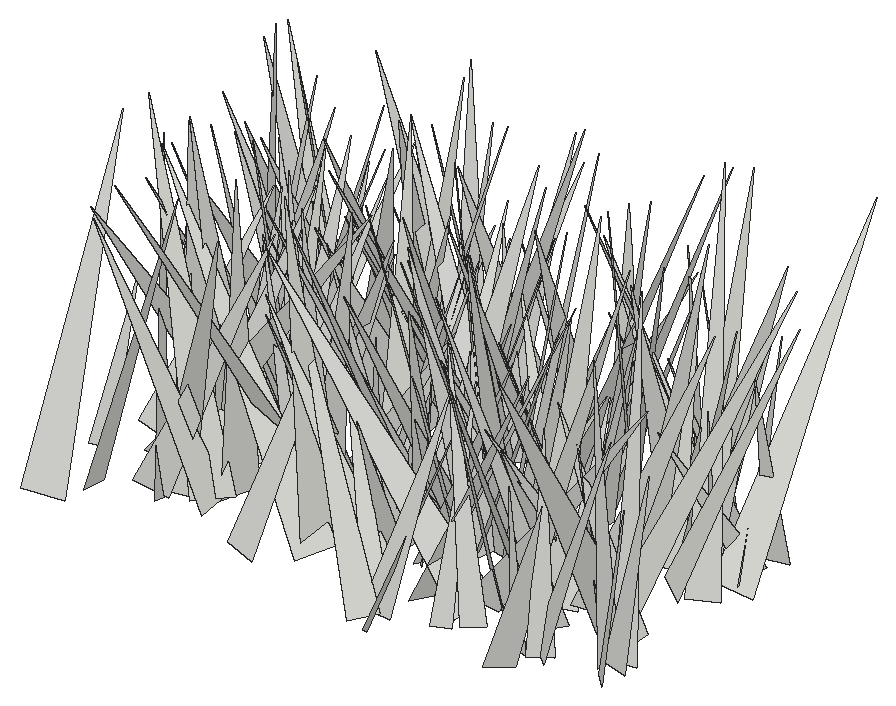
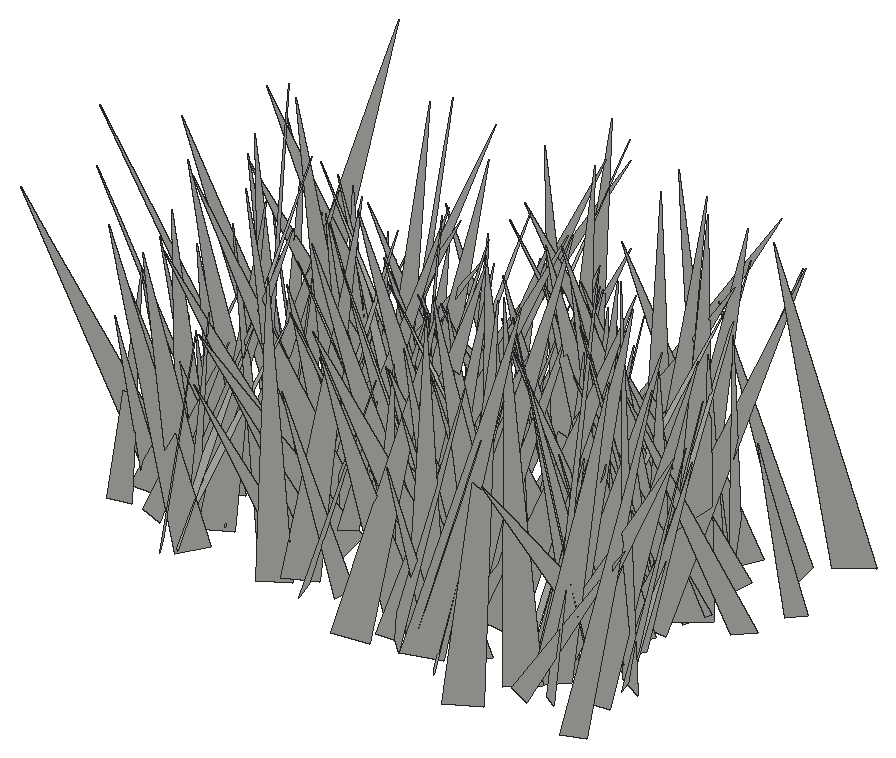
# SketchUp Ruby script. Lengths in inches.
U = 1.inch
M = Sketchup.active_model
def pt(a) = Geom::Point3d.new(a.map { |v| v * U })
def face(e, loops, mat)
  f = e.add_face(loops[0].map { |a| pt(a) })
  loops[1..].each { |l| e.add_face(l.map { |a| pt(a) }).erase! }
  f.material = f.back_material = mat if mat
  f
end
# faces: each face lists its corners as indices into pts; further lists are holes
def faces(e, pts, list, mat = nil) = list.each { |f| face(e, (f[0].is_a?(Array) ? f : [f]).map { |l| l.map { |i| pts[i] } }, mat) }
# xy, xz, yz: faces in a plane at the given z, y or x. An outline is a flat list of corners, or four numbers for a rectangle; further outlines are holes
def ring(l) = l.size == 4 ? [[l[0], l[1]], [l[2], l[1]], [l[2], l[3]], [l[0], l[3]]] : l.each_slice(2).to_a
def flat(e, list, mat, &to3) = list.each { |f| face(e, (f[0].is_a?(Array) ? f : [f]).map { |l| ring(l).map { |u, v| to3.(u, v) } }, mat) }
def xy(e, z, list, mat = nil) = flat(e, list, mat) { |x, y| [x, y, z] }
def xz(e, y, list, mat = nil) = flat(e, list, mat) { |x, z| [x, y, z] }
def yz(e, x, list, mat = nil) = flat(e, list, mat) { |y, z| [x, y, z] }
def lines(e, pts, list) = list.each { |a, b| e.add_line(pt(pts[a]), pt(pts[b])) }
# prism: a flat outline (further loops are holes) pulled along v
def prism(e, loops, v, mat = nil)
  f = face(e, loops, mat); d = Geom::Vector3d.new(v.map { |x| x * U })
  f.pushpull(f.normal.samedirection?(d) ? d.length : -d.length)
end
def box(e, o, s, mat = nil) = prism(e, [[o, [o[0] + s[0], o[1], o[2]], [o[0] + s[0], o[1] + s[1], o[2]], [o[0], o[1] + s[1], o[2]]]], [0, 0, s[2]], mat)
def at(x, y, z, deg = 0) = Geom::Transformation.translation(pt([x, y, z])) * Geom::Transformation.rotation(ORIGIN, Z_AXIS, deg.degrees)
def axes(o, x, y, z) = Geom::Transformation.new([*x, 0, *y, 0, *z, 0, *pt(o).to_a, 1])
def part(name) = M.definitions.add(name)
# library, detail: a bought-in or finely detailed component or shape, given as its bounding box
def library(name, o, s) = part(name).tap { |d| box(d.entities, o, s) }
def detail(e, o, s) = box(e.add_group.entities, o, s)
def put(e, d, t, mat = nil) = e.add_instance(d, t).tap { |i| i.material = mat if mat }
def group(e, t, mat = nil) = e.add_group.tap { |g| g.transformation = t; g.material = mat if mat }.entities
root = M.entities
c1 = part("fur_instance\#9")
p = [[0.8125,0,1.79],[0.67,-0.02,1.48],[0,-0.11,0],[0,0.11,0]]
faces(c1.entities,p,[[0,1,2,3]])
put(root,c1,axes([541.4,84.6,-21.86],[-0.86303,4.80618,1.97762],[4.83833,1.47497,-1.47315],[1.8976,-1.57489,4.65553]))
put(root,c1,axes([547.29,85.66,-21.86],[-0.48209,-3.49328,1.24378],[-3.69826,0.54426,0.09516],[0.26993,1.21786,3.5251]))
put(root,c1,axes([549.19,89.3125,-21.86],[4.52461,-6.7861,0.00105],[-6.53347,-4.35651,-2.20405],[-1.83437,-1.22185,7.85273]))
put(root,c1,axes([548.17,85.83,-21.66],[3.55889,4.26793,1.49162],[4.48448,-3.09137,-1.85436],[0.57409,-2.30955,5.23854]))
put(root,c1,axes([541.21,84.09,-21.86],[-2.13966,5.92839,0.3544],[5.56639,1.87053,2.31645],[-2.07043,-1.09766,5.86157]))
put(root,c1,axes([544.48,88.09,-21.86],[-3.66849,-5.82093,1.22872],[-5.44278,3.86666,2.06783],[2.40191,-0.1285,6.56241]))
put(root,c1,axes([542.1,83.03,-21.66],[3.66299,2.22216,0.32756],[1.7102,-3.16536,2.34915],[-1.4562,1.87225,3.58288]))
put(root,c1,axes([526.11,83.92,-21.86],[-2.77927,7.20298,1.80131],[7.21654,3.07297,-1.15349],[1.74623,-1.2353,7.63392]))
put(root,c1,axes([543.86,87.31,-21.86],[-7.78216,2.50032,0.23977],[2.4235,7.26917,2.85602],[-0.66011,-2.78901,7.65877]))
put(root,c1,axes([531.58,87.31,-21.86],[-6.5147,0.26004,1.16019],[0.55336,6.38259,1.67669],[1.05235,-1.74639,6.3006]))
put(root,c1,axes([529.17,88.22,-21.66],[-0.1774,-7.7519,1.13116],[-7.17611,0.61466,3.08685],[3.14245,0.96602,7.113]))
put(root,c1,axes([548.23,85.8125,-21.86],[-2.69115,3.5868,1.84623],[3.86426,2.92918,-0.05799],[1.15809,-1.43902,4.48375]))
put(root,c1,axes([540.28,86.5,-21.66],[-4.33976,4.07233,1.17149],[4.17045,3.80756,2.21352],[-0.75076,-2.38923,5.52429]))
put(root,c1,axes([539.65,87.96,-21.66],[4.21418,-1.38432,0.79636],[-0.98829,-4.02576,-1.76817],[-1.25452,-1.47878,4.06808]))
put(root,c1,axes([551.07,85.82,-21.86],[-2.22453,-2.28888,1.93607],[-2.6411,2.63697,0.08289],[1.41842,1.32035,3.19071]))
put(root,c1,axes([536.79,87.33,-21.86],[4.88048,-6.02987,2.56967],[-6.14977,-5.32095,-0.80587],[-2.26779,1.4525,7.7155]))
put(root,c1,axes([541.1875,84.92,-21.66],[-1.53438,4.71255,0.03454],[4.47921,1.44703,1.55125],[-1.46492,-0.51147,4.70702]))
put(root,c1,axes([550.89,86.85,-21.86],[0.22976,-4.49295,1.68417],[-4.67204,0.17468,1.10336],[1.09322,1.69077,4.36142]))
put(root,c1,axes([546.88,87.34,-21.66],[-4.74845,-6.02691,1.04144],[-6.05438,4.44477,-1.88271],[-0.8676,1.96887,7.4382]))
put(root,c1,axes([536.43,88.92,-21.86],[-2.23996,-8.03771,0.28468],[-7.44594,1.96073,-3.22749],[-3.04036,1.11981,7.69451]))
put(root,c1,axes([542.23,88.01,-21.66],[-3.30387,-7.05223,0.96215],[-6.92829,2.9435,-2.21582],[-1.63048,1.78244,7.4659]))
put(root,c1,axes([527.14,85.67,-21.86],[6.05583,0.88682,1.38397],[0.67013,-6.15634,1.01257],[-1.50092,0.82941,6.03608]))
put(root,c1,axes([529.21,86.48,-21.66],[3.36914,-5.54095,2.01408],[-5.73384,-2.5398,2.60427],[1.37175,2.99283,5.93894]))
put(root,c1,axes([545.06,85.8125,-21.66],[-1.00856,5.27208,0.80529],[5.17147,0.76643,1.45913],[-1.30357,-1.0384,5.16556]))
put(root,c1,axes([544.16,85,-21.66],[-4.2837,1.86088,0.37109],[1.60299,4.03921,-1.75094],[1.01537,1.47394,4.32979]))
put(root,c1,axes([547.48,84.29,-21.86],[7.73551,0.03019,2.73159],[-1.01366,-7.58581,2.95441],[-2.53672,3.12332,7.14916]))
put(root,c1,axes([536.48,87.87,-21.86],[0.04247,-7.07988,2.41623],[-7.48051,-0.06275,-0.05238],[-0.06984,2.41579,7.07981]))
put(root,c1,axes([542,86.55,-21.86],[5.54197,-0.978,0.47716],[-1.05474,-5.437,1.10644],[-0.26776,1.17482,5.51777]))
put(root,c1,axes([531.82,88.54,-21.86],[6.66168,-2.88093,2.18206],[-2.80757,-7.00677,-0.67958],[-2.27567,0.211,7.22605]))
put(root,c1,axes([550.48,87.03,-21.86],[-5.81537,-0.03657,1.70774],[-0.23888,6.01751,-0.6846],[1.69135,0.72416,5.77505]))
put(root,c1,axes([537.98,88.29,-21.86],[-2.3451,-4.39084,0.71964],[-4.31416,2.04482,-1.58228],[-1.08875,1.35503,4.71968]))
put(root,c1,axes([531.46,87.33,-21.66],[-4.16616,6.68617,2.08588],[7.00105,3.90518,1.46546],[-0.20279,-2.54114,7.74043]))
put(root,c1,axes([536.8,86.8125,-21.86],[-4.02573,7.19257,0.41274],[6.48293,3.4104,3.80141],[-3.14246,-2.17854,7.31361]))
put(root,c1,axes([539.29,91,-21.66],[-6.65977,-5.09555,0.25994],[-4.96209,6.56797,1.61994],[1.1874,-1.13219,8.22757]))
put(root,c1,axes([549.32,88.21,-21.86],[-3.81411,-2.18756,1.38745],[-2.30966,3.98998,-0.05835],[1.17299,0.74331,4.39652]))
put(root,c1,axes([544.01,87.63,-21.86],[4.55,-4.60588,0.41001],[-4.16176,-3.82822,3.1795],[2.01545,2.49305,5.6398]))
put(root,c1,axes([534.52,85.09,-21.86],[2.76635,7.35948,0.05567],[7.35952,-2.76581,-0.07342],[0.04914,-0.07794,7.86188]))
put(root,c1,axes([535.28,89.14,-21.86],[0.67729,-7.55263,2.0847],[-7.70125,-0.25666,1.57216],[1.44182,2.17688,7.41817]))
put(root,c1,axes([547.53,87.68,-21.66],[-2.26256,-5.81888,2.33683],[-5.71547,0.89178,-3.31322],[-2.57945,3.12805,5.2916]))
put(root,c1,axes([550.29,88.94,-21.86],[-5.1344,0.67452,1.09766],[0.89094,5.11676,1.02317],[0.93062,-1.17714,5.07643]))
put(root,c1,axes([536.19,90.23,-21.86],[0.26999,-5.16111,0.17986],[-5.16087,-0.27616,-0.17741],[-0.18667,0.17024,5.16512]))
put(root,c1,axes([529.74,86.41,-21.86],[-6.50203,-1.48304,1.94789],[-2.15091,6.10063,-2.53495],[1.1693,2.97539,6.16846]))
put(root,c1,axes([530.19,87.12,-21.86],[0.38602,5.6901,1.15392],[5.67114,-0.61727,1.14668],[-1.24374,-1.04858,5.58671]))
put(root,c1,axes([525.49,88.11,-21.86],[-1.54021,3.23682,1.39983],[3.28512,1.87235,-0.71486],[1.28237,-0.90889,3.51258]))
put(root,c1,axes([529.09,92.55,-21.66],[4.10096,-6.21113,0.1393],[-5.64172,-3.79303,-3.03306],[-2.60165,-1.56533,6.79681]))
put(root,c1,axes([529.95,89.82,-21.86],[3.24769,-2.54753,0.32293],[-2.51539,-3.26077,-0.4265],[-0.51676,-0.13836,4.10555]))
put(root,c1,axes([528.28,88.55,-21.66],[5.80573,-6.03364,0.3689],[-5.4436,-4.99608,3.95649],[2.62833,2.98023,7.37953]))
put(root,c1,axes([535.4,90.61,-21.66],[-3.59225,-3.71334,1.0598],[-3.39845,3.72735,1.54069],[1.83374,-0.36648,4.93148]))
put(root,c1,axes([535.61,87.4375,-21.66],[-5.65883,0.17912,0.29432],[0.09895,5.4838,-1.43499],[0.33003,1.4272,5.47679]))
put(root,c1,axes([542.875,90.79,-21.86],[-0.69616,-7.71222,1.47846],[-7.81205,0.83092,0.65597],[0.79755,1.40715,7.71575]))
put(root,c1,axes([544.75,91.21,-21.86],[3.43107,-2.8474,0.0502],[-2.64084,-3.2106,-1.6126],[-1.06592,-1.21113,4.15686]))
put(root,c1,axes([530.47,90.54,-21.66],[6.98287,-2.99298,2.96369],[-2.61118,-7.57832,-1.50091],[-3.30502,-0.33623,7.44753]))
put(root,c1,axes([530.91,87.93,-21.86],[-2.71022,2.78687,0.60598],[2.7235,2.77712,-0.59105],[0.8464,-0.01233,3.84222]))
put(root,c1,axes([545.93,91.77,-21.86],[-4.54437,-2.07997,0.71062],[-1.49312,4.11891,2.50752],[1.61302,-2.04715,4.32318]))
put(root,c1,axes([541.79,90.64,-21.86],[-6.14349,2.42883,3.06477],[3.31416,6.26335,1.67969],[2.07568,-2.81172,6.38908]))
put(root,c1,axes([542.3,88.83,-21.66],[-6.0406,-4.0795,1.11122],[-4.22494,5.74856,-1.86274],[-0.16426,2.16279,7.04708]))
put(root,c1,axes([543.93,89.92,-21.86],[4.55769,0.07164,0.01251],[0.0727,-4.46545,-0.91231],[0.00209,-0.91239,4.46602]))
put(root,c1,axes([550.91,87.32,-21.86],[0.5538,7.06628,1.29605],[7.05626,-0.7792,1.23321],[-1.34954,-1.17443,6.97985]))
put(root,c1,axes([540.36,88.83,-21.86],[4.95013,-1.23925,0.4471],[-1.29852,-4.88303,0.8422],[-0.22245,0.9272,5.03291]))
put(root,c1,axes([539.81,91.72,-21.86],[0.04578,-6.29285,0.19538],[-6.21134,-0.07706,-1.02644],[-1.02831,0.18529,6.20874]))
put(root,c1,axes([546.54,90.17,-21.66],[-1.84266,-5.86998,0.99209],[-5.21002,1.08759,-3.24178],[-2.88039,1.78795,5.22904]))
put(root,c1,axes([528.28,90.92,-21.86],[5.79688,-5.3049,1.7816],[-5.31494,-6.02201,-0.63769],[-1.75142,0.71643,7.83193]))
put(root,c1,axes([540.96,89.09,-21.86],[6.16739,3.42449,0.19717],[3.4017,-6.05394,-1.25736],[0.441,-1.19388,6.94138]))
put(root,c1,axes([540.34,88.57,-21.86],[2.54415,2.86578,1.34064],[2.68524,-2.86561,1.02977],[-1.67317,-0.2414,3.6912]))
put(root,c1,axes([539.1875,89.2,-21.86],[-5.93557,-1.05009,0.32847],[-1.08922,5.86272,-0.94003],[0.15548,0.98355,5.95399]))
put(root,c1,axes([538.43,91.43,-21.86],[5.5268,-1.95543,1.04999],[-1.67194,-5.52102,-1.48142],[-1.45972,-1.07995,5.67227]))
put(root,c1,axes([529.57,88.59,-21.86],[-2.26569,5.88907,2.62757],[5.5866,3.18358,-2.31806],[3.22106,-1.37923,5.86866]))
put(root,c1,axes([541.58,90.53,-21.66],[6.21728,1.67139,0.47713],[1.73743,-6.02723,-1.52629],[-0.05031,-1.59834,6.25448]))
put(root,c1,axes([533.58,90.79,-21.86],[-5.94217,-4.1756,0.21971],[-4.13273,5.80684,-1.41225],[-0.63601,1.27993,7.12394]))
put(root,c1,axes([547.49,89.74,-21.86],[4.70932,-5.02611,1.74089],[-5.27526,-4.11549,2.38842],[0.68127,2.87596,6.46026]))
put(root,c1,axes([545.52,89.51,-21.86],[-0.77106,7.66776,2.67234],[8.04873,1.0768,-0.76736],[1.07416,-2.56446,7.66813]))
put(root,c1,axes([534.67,88.9,-21.86],[-6.42625,-2.81034,1.42452],[-3.14557,5.90814,-2.53441],[0.18076,2.90169,6.53999]))
put(root,c1,axes([546.68,89.22,-21.86],[-1.99149,3.68652,0.84504],[3.6319,2.13053,-0.73532],[1.05538,-0.37542,4.12502]))
put(root,c1,axes([535,90.3125,-21.66],[2.54302,-4.52945,1.06711],[-4.23804,-1.75205,2.66287],[1.92189,2.12978,4.46004]))
put(root,c1,axes([533.24,88.83,-21.66],[5.43285,-3.6045,3.64876],[-4.74936,-5.54221,1.59663],[-1.93634,3.48041,6.32132]))
put(root,c1,axes([530.24,90.42,-21.86],[-3.99726,2.72851,1.81883],[2.89094,4.28575,-0.07581],[1.5477,-0.9584,4.83912]))
put(root,c1,axes([544.84,92.68,-21.86],[-3.72414,-4.2026,0.59605],[-4.10843,3.76818,0.89886],[1.06672,-0.15915,5.54285]))
put(root,c1,axes([530.14,90.67,-21.86],[3.39124,-4.48702,2.29298],[-4.9912,-3.37077,0.78574],[-0.69206,2.32297,5.56924]))
put(root,c1,axes([538.04,89.09,-21.86],[3.94824,4.29759,0.4959],[4.2386,-3.97723,0.72087],[-0.86569,0.12707,5.79122]))
put(root,c1,axes([539.92,91.44,-21.86],[-2.80028,2.24736,2.49663],[2.73085,3.4158,-0.01176],[1.95607,-1.55147,3.59055]))
put(root,c1,axes([533.42,90.44,-21.86],[-0.70822,-5.57958,3.0516],[-6.3293,0.31925,-0.88519],[-0.61961,3.1164,5.55425]))
put(root,c1,axes([541.1,92.38,-21.86],[-4.24041,-4.62675,0.86788],[-4.65391,4.29598,0.16351],[0.70788,0.52807,6.27385]))
put(root,c1,axes([530.07,89.39,-21.86],[7.54644,-1.30772,2.23251],[-1.88035,-7.50036,1.96263],[-1.77721,2.38276,7.40318]))
put(root,c1,axes([535.13,89.65,-21.86],[-5.60196,1.71083,0.59088],[1.59688,5.57635,-1.00614],[0.85208,0.79713,5.77032]))
put(root,c1,axes([532.51,89.95,-21.86],[0.3651,6.79595,1.75212],[7.01816,-0.34958,-0.10649],[0.01583,-1.75528,6.80491]))
put(root,c1,axes([543.93,88.76,-21.66],[4.5947,4.98178,1.41698],[4.55399,-4.78808,2.06705],[-2.46722,0.43974,6.4542]))
put(root,c1,axes([527.27,95.85,-21.66],[-5.00279,-6.48805,0.18943],[-5.66686,4.48249,3.86684],[3.16501,-2.22958,7.22289]))
put(root,c1,axes([533.22,90.75,-21.86],[4.31663,-3.25233,1.38409],[-3.53279,-4.03972,1.52536],[-0.11299,2.05661,5.185]))
put(root,c1,axes([529.62,91.57,-21.86],[-4.67685,-1.64881,1.07356],[-1.71505,4.77313,-0.14071],[0.96421,0.49258,4.95698]))
put(root,c1,axes([533,91.27,-21.86],[-6.02179,2.8816,2.13168],[3.11245,6.27078,0.31555],[1.77772,-1.21792,6.66828]))
put(root,c1,axes([532.36,91.91,-21.86],[5.34451,-3.5502,0.35957],[-3.55754,-5.25077,1.03462],[0.27778,1.05952,6.33224]))
put(root,c1,axes([535.5,91.92,-21.86],[3.51099,-0.42801,1.09439],[-0.295,-3.65871,-0.48452],[-1.13748,-0.37227,3.50364]))
put(root,c1,axes([528.19,90.62,-21.86],[3.23121,-4.00646,1.7311],[-4.24322,-2.37965,2.41277],[1.02152,2.78831,4.54653]))
put(root,c1,axes([548.87,89.78,-21.86],[0.48963,4.22721,0.04806],[3.94805,-0.47454,1.51627],[-1.51146,0.12987,3.97618]))
put(root,c1,axes([530.78,90.66,-21.86],[-2.41477,3.3901,0.55663],[3.41153,2.44646,-0.10002],[0.40504,-0.3947,4.161]))
put(root,c1,axes([526.21,90.32,-21.86],[-0.28996,5.60424,1.15409],[5.32871,0.68543,-1.98963],[2.08431,-0.97272,5.24719]))
put(root,c1,axes([542.34,92.76,-21.86],[-0.32261,-5.78503,1.74562],[-5.69921,0.87225,1.8374],[2.00818,1.5461,5.49497]))
put(root,c1,axes([542.14,91.625,-21.66],[2.38056,3.51502,0.37387],[3.33138,-2.08023,-1.65431],[1.18197,-1.21634,3.90969]))
put(root,c1,axes([528.64,93.6,-21.66],[2.77166,-6.45652,0.14972],[-5.9267,-2.47813,2.8503],[2.56578,1.25036,6.42219]))
put(root,c1,axes([542.96,93.71,-21.86],[-1.61608,-6.86234,1.14057],[-6.89566,1.42577,-1.19223],[-0.91789,1.37106,6.94853]))
put(root,c1,axes([548.35,90.65,-21.86],[3.48936,7.09192,0.65775],[6.9322,-3.21357,-2.12629],[1.63479,-1.51038,7.61247]))
put(root,c1,axes([546.23,94.0625,-21.66],[-5.2101,-5.93708,2.74108],[-5.84341,5.80017,1.45611],[2.93548,1.00834,7.76362]))
put(root,c1,axes([539.77,94.89,-21.86],[-1.57704,-7.74459,0.50786],[-7.45096,1.36569,-2.31124],[-2.17253,0.93802,7.55804]))
put(root,c1,axes([532.09,95.49,-21.66],[-3.9218,-4.42687,0.35438],[-4.07666,3.77609,2.05553],[1.7617,-1.11678,5.54549]))
put(root,c1,axes([542.36,92.29,-21.66],[-3.42492,-4.02626,1.68032],[-4.34426,2.9504,-1.78518],[-0.40205,2.41841,4.97534]))
put(root,c1,axes([530.37,90.37,-21.66],[3.83849,6.3713,1.10198],[6.13828,-3.99344,1.70758],[-2.03209,-0.02789,7.23959]))
put(root,c1,axes([536.67,91.61,-21.86],[-6.2785,3.87073,1.88034],[3.7817,6.55006,-0.85632],[2.05354,-0.22787,7.32591]))
put(root,c1,axes([539.72,93.34,-21.86],[-5.07554,-4.81191,2.50581],[-5.17107,5.32884,-0.24106],[1.64121,1.90882,6.98981]))
put(root,c1,axes([534.58,96.33,-21.66],[-6.04066,-0.63869,2.51357],[0.73038,5.69455,3.20222],[2.48847,-3.22176,5.16172]))
put(root,c1,axes([538.41,92.17,-21.66],[-1.59502,6.99566,2.35908],[7.02793,2.17795,-1.70682],[2.26111,-1.83463,6.96922]))
put(root,c1,axes([531.01,94.14,-21.86],[1.01091,-5.94061,2.30759],[-6.04054,-1.63799,-1.57056],[-2.03168,1.91413,5.81775]))
put(root,c1,axes([538.34,95.24,-21.66],[-2.23247,-5.83337,0.18602],[-5.6892,2.13065,-1.46288],[-1.30221,0.692,6.07224]))
put(root,c1,axes([543.93,89.1875,-21.66],[4.35175,7.0169,0.44581],[6.16578,-4.0605,3.72408],[-3.37917,1.6275,7.36925]))
put(root,c1,axes([528.36,94,-21.86],[-4.20728,0.83557,0.99678],[1.00115,4.23485,0.67581],[0.83033,-0.87227,4.23588]))
put(root,c1,axes([548.8125,92.85,-21.86],[3.72746,5.46093,0.78491],[5.42353,-3.45332,-1.72965],[1.01153,-1.60767,6.38153]))
put(root,c1,axes([536.39,92.61,-21.86],[4.3038,1.80689,1.01933],[1.67441,-4.41138,0.75005],[-1.22483,0.31842,4.60705]))
put(root,c1,axes([536.82,90.23,-21.86],[5.37795,5.75,0.47067],[5.40496,-5.24661,2.33794],[-2.01755,1.27162,7.51791]))
put(root,c1,axes([533.23,96.03,-21.66],[1.95168,-6.84621,1.26966],[-6.52036,-2.2596,-2.16121],[-2.44285,0.56154,6.78298]))
put(root,c1,axes([550.52,95.75,-21.86],[2.70067,-3.13661,0.88183],[-2.51329,-2.73437,-2.02883],[-2.07348,-0.77102,3.60774]))
put(root,c1,axes([538.42,93.08,-21.86],[5.52496,2.9641,0.73245],[3.00682,-5.54515,-0.24054],[-0.53047,-0.55942,6.26523]))
put(root,c1,axes([547.29,93.05,-21.86],[6.61649,-1.70465,2.3436],[-2.13195,-6.81989,1.0584],[-1.96294,1.66119,6.75008]))
put(root,c1,axes([537.36,94.08,-21.86],[4.26673,-0.51352,0.23406],[-0.5171,-4.27238,0.05285],[-0.22604,0.08052,4.29719]))
put(root,c1,axes([529.9375,92.42,-21.86],[6.18202,1.83786,0.77531],[1.68935,-6.16651,1.14736],[-1.06062,0.8903,6.34654]))
put(root,c1,axes([543.64,94.38,-21.86],[3.4231,3.63538,1.50249],[3.93251,-3.11512,-1.42212],[0.09387,-2.06666,4.78656]))
put(root,c1,axes([550,93.91,-21.86],[1.56672,2.93333,1.48069],[3.11219,-1.85095,0.37383],[-1.05412,-1.105,3.30444]))
put(root,c1,axes([540.23,93.57,-21.66],[-4.97351,5.86998,1.15657],[5.9442,4.67754,1.82131],[-0.6788,-2.04794,7.47498]))
put(root,c1,axes([536.03,97.07,-21.86],[-0.13701,-6.93499,0.01519],[-6.899,0.13785,0.70555],[0.70571,0.00117,6.90036]))
put(root,c1,axes([527.26,98.01,-21.86],[5.40671,-4.03304,0.21931],[-3.53675,-4.90438,-2.9974],[-1.95061,-2.2864,6.04264]))
put(root,c1,axes([534.26,97.77,-21.86],[1.01288,-8.11783,0.06805],[-8.08119,-1.01477,-0.77093],[-0.77341,-0.02823,8.14437]))
put(root,c1,axes([533.87,95.18,-21.86],[5.79925,-1.98106,0.58125],[-1.98372,-5.82701,-0.06806],[-0.57211,0.1232,6.12791]))
put(root,c1,axes([531.31,93.5625,-21.86],[4.10356,-2.98524,2.70877],[-3.77942,-4.1935,1.10399],[-1.40181,2.56732,4.95298]))
put(root,c1,axes([546.34,96.45,-21.86],[4.71186,-4.25626,1.34995],[-4.06485,-4.9009,-1.26409],[-1.848,-0.07223,6.22249]))
put(root,c1,axes([538.38,91.99,-21.66],[-4.13598,4.27474,0.09369],[4.07434,3.97972,-1.71759],[1.29691,1.13001,5.6947]))
put(root,c1,axes([548.95,94.76,-21.86],[-0.57371,3.97778,1.97621],[4.19128,1.14438,-1.08668],[1.47014,-1.71025,3.86924]))
put(root,c1,axes([547.97,94.69,-21.86],[5.31059,0.52385,1.16283],[0.52648,-5.43598,0.04446],[-1.16164,-0.06886,5.33618]))
put(root,c1,axes([547.69,94,-21.86],[-2.00411,5.21831,1.67163],[5.38658,2.20263,-0.41796],[1.00489,-1.39973,5.57427]))
put(root,c1,axes([541.375,97.71,-21.66],[6.17469,-3.94346,0.96595],[-3.5616,-6.10514,-2.15707],[-1.94909,-1.33681,7.00177]))
put(root,c1,axes([542.65,93.02,-21.86],[8.13769,0.92636,1.08085],[0.65484,-8.00564,1.93114],[-1.26395,1.81658,7.95932]))
put(root,c1,axes([543.93,94.76,-21.86],[7.00703,0.38351,2.14023],[0.30488,-7.32356,0.31416],[-2.15283,0.21111,7.01048]))
put(root,c1,axes([531.06,94.67,-21.86],[-4.50468,1.1443,0.55643],[1.12699,4.53841,-0.20945],[0.5907,0.0676,4.64302]))
put(root,c1,axes([546.5,96.29,-21.86],[0.84418,-3.62493,0.18375],[-3.45271,-0.74384,1.18829],[1.11924,0.43944,3.52714]))
put(root,c1,axes([541.92,94.43,-21.86],[-3.84574,2.31871,0.01808],[2.31862,3.84577,-0.02193],[0.02681,0.00945,4.49062]))
put(root,c1,axes([538,94.14,-21.86],[6.16496,0.12051,1.82007],[-0.27856,-6.27765,1.3592],[-1.80266,1.38221,6.01447]))
put(root,c1,axes([526.93,96.15,-21.86],[4.42565,6.01002,3.52258],[6.87552,-4.43985,-1.06317],[-1.12079,-3.50468,7.38759]))
put(root,c1,axes([527.17,96.04,-21.86],[-4.98874,-1.77944,1.14235],[-1.81158,5.1064,0.04294],[1.09068,0.3424,5.29642]))
put(root,c1,axes([547.59,96.73,-21.66],[-5.95975,2.47486,1.75961],[2.91321,5.75356,1.77469],[0.85695,-2.34763,6.20435]))
put(root,c1,axes([546.71,98.45,-21.66],[-5.73536,-5.62008,0.65862],[-5.46135,5.74328,1.44982],[1.48081,-0.58562,7.89796]))
put(root,c1,axes([527.89,95.42,-21.86],[2.6257,3.60497,0.95618],[3.72031,-2.44904,-0.98281],[0.26337,-1.34567,4.35019]))
put(root,c1,axes([548.92,94.54,-21.86],[4.55494,-1.38322,1.77977],[-1.90749,-4.50337,1.38185],[-1.20098,1.9065,4.55536]))
put(root,c1,axes([530.1,96.78,-21.86],[2.50523,-6.92108,2.84903],[-7.08461,-3.16179,-1.45116],[-2.41383,2.09672,7.21607]))
put(root,c1,axes([550.27,92.89,-21.86],[0.30584,8.28043,0.48557],[7.987,-0.4251,2.21855],[-2.2381,-0.38549,7.98355]))
put(root,c1,axes([543.54,97.03,-21.86],[6.22131,1.299,1.34326],[1.60809,-6.10017,-1.54868],[-0.95174,-1.81575,6.1639]))
put(root,c1,axes([550.56,96.96,-21.86],[1.07632,-4.38935,0.89904],[-4.4763,-1.09335,0.02097],[-0.19334,0.87825,4.51934]))
put(root,c1,axes([535.05,94.27,-21.86],[-6.71814,2.72987,2.53139],[2.23652,7.13443,-1.75826],[2.97626,0.8008,7.03521]))
put(root,c1,axes([547.55,97.08,-21.86],[-3.79986,-3.34827,0.10157],[-3.34083,3.7767,-0.4853],[-0.24505,0.43103,5.04126]))
put(root,c1,axes([529.85,97.55,-21.86],[2.72704,-3.27265,0.76108],[-3.17295,-2.83078,-0.80329],[-1.10537,0.05182,4.1835]))
put(root,c1,axes([530.11,98.55,-21.86],[2.36593,-6.95857,0.28973],[-6.83072,-2.25873,1.53056],[1.359,0.76137,7.18865]))
put(root,c1,axes([548.94,97.08,-21.86],[-0.5806,-4.0301,0.94816],[-3.96701,0.26756,-1.29192],[-1.18471,1.07913,3.86131]))
put(root,c1,axes([528.41,99.08,-21.66],[-4.91582,-6.36103,2.07601],[-5.8042,5.33544,2.60426],[3.32923,-0.09063,7.60565]))
put(root,c1,axes([550.77,94.8,-21.86],[-4.5247,0.14497,1.56827],[-0.47946,4.4174,-1.79167],[1.5002,1.84904,4.15738]))
put(root,c1,axes([527.79,97.24,-21.66],[5.79589,4.16761,1.50359],[4.42839,-5.37215,-2.17978],[0.13803,-2.64446,6.79779]))
put(root,c1,axes([538.25,96.77,-21.86],[-1.45922,4.42701,2.15741],[4.90506,1.50733,0.22462],[0.43952,-2.12407,4.65589]))
put(root,c1,axes([536.93,95.7,-21.86],[7.47756,-1.51643,1.55812],[-1.8154,-7.42558,1.48539],[-1.19651,1.78955,7.48379]))
put(root,c1,axes([541.37,94.63,-21.66],[5.52796,-0.81869,0.7417],[-1.07099,-4.89962,2.57397],[-0.27083,2.66498,4.96017]))
put(root,c1,axes([530.12,96.66,-21.66],[-1.81659,5.58818,1.87966],[5.39696,0.78429,2.88421],[-2.37355,-2.49359,5.11948]))
put(root,c1,axes([536.82,94.81,-21.86],[-3.66435,5.27166,1.90181],[4.6134,4.12758,-2.55233],[3.18179,0.08644,5.89097]))
put(root,c1,axes([543.68,93.9,-21.86],[7.3603,1.92647,1.4977],[1.22652,-7.03518,3.02165],[-2.10951,2.63124,6.98247]))
put(root,c1,axes([536.375,98.86,-21.86],[1.81992,-3.21241,0.00061],[-3.09433,-1.75321,-0.99152],[-0.86298,-0.48823,3.55649]))
put(root,c1,axes([535.88,95.55,-21.86],[-6.0255,1.4926,2.28597],[0.94971,6.33899,-1.63567],[2.5596,1.16168,5.98825]))
put(root,c1,axes([539.63,97.25,-21.86],[4.04534,-0.8517,0.30361],[-0.87788,-4.03293,0.38361],[-0.21657,0.43867,4.11619]))
put(root,c1,axes([526.28,100.37,-21.86],[6.25747,-1.85529,1.59771],[-1.00282,-5.94215,-2.97253],[-2.23363,-2.52972,5.81052]))
put(root,c1,axes([529.46,94.2,-21.66],[-3.68567,4.23937,0.30212],[3.60627,3.33103,-2.74713],[2.24908,1.60613,4.89997]))
put(root,c1,axes([550.63,94.21,-21.86],[-1.16046,8.00046,0.20395],[7.87345,1.17823,-1.41992],[1.43448,0.00519,7.95851]))
put(root,c1,axes([540.95,98.03,-21.86],[-4.66141,-1.64687,0.68606],[-1.65466,4.70851,0.06011],[0.66704,0.1713,4.94341]))
put(root,c1,axes([547.46,96.5,-21.66],[-5.30333,-1.20318,1.41609],[-1.56427,5.2022,-1.4382],[1.00301,1.75149,5.24448]))
put(root,c1,axes([537.36,99.74,-21.86],[2.99002,-5.93259,1.12286],[-5.76165,-3.17812,-1.449],[-1.8055,0.31717,6.48354]))
put(root,c1,axes([533.375,99.78,-21.86],[-4.0085,-3.44331,0.94309],[-3.06456,4.04605,1.74695],[1.83147,-0.76613,4.98725]))
put(root,c1,axes([542.27,98.13,-21.86],[2.8988,-5.16102,2.16058],[-5.5292,-3.01461,0.21733],[-0.85564,1.9958,5.91539]))
put(root,c1,axes([536.31,96.73,-21.86],[-5.43034,-1.89464,0.64767],[-1.9986,5.01546,-2.08529],[-0.12137,2.18018,5.36002]))
put(root,c1,axes([529.375,97.79,-21.86],[-5.93712,3.87569,1.72238],[4.1151,5.9813,0.72589],[1.02637,-1.56207,7.0529]))
put(root,c1,axes([543.41,95.96,-21.86],[4.47299,1.54799,0.88013],[1.09405,-4.26651,1.94385],[-1.40498,1.60599,4.31572]))
put(root,c1,axes([532.37,98.24,-21.66],[1.52627,-4.48364,1.33128],[-4.39877,-0.90019,2.01128],[1.58937,1.81423,4.28804]))
put(root,c1,axes([545.87,98.46,-21.66],[3.29636,-5.4576,1.30622],[-5.51274,-2.86598,1.93739],[1.04942,2.08768,6.07437]))
put(root,c1,axes([530.95,101.08,-21.86],[6.44625,-4.17663,0.34492],[-3.99481,-6.31514,-1.81045],[-1.26676,-1.33867,7.46462]))
put(root,c1,axes([529.78,99.18,-21.86],[-0.38653,-3.78857,0.47263],[-3.40937,0.1287,-1.7566],[-1.71837,0.59684,3.37891]))
put(root,c1,axes([534.21,99.43,-21.66],[4.0303,-5.81988,3.12764],[-5.66664,-4.92868,-1.86917],[-3.39741,1.31665,6.82792]))
put(root,c1,axes([547.42,96.55,-21.86],[-6.19625,3.45387,1.64148],[3.0912,6.3638,-1.72156],[2.25127,0.76815,6.88178]))
put(root,c1,axes([547.28,98.53,-21.86],[-4.18009,-2.38384,1.39005],[-2.61185,4.23208,-0.59649],[0.8906,1.22265,4.77494]))
put(root,c1,axes([535.12,98.05,-21.86],[-2.11891,6.73628,2.3501],[7.12334,2.13432,0.30482],[0.39806,-2.33612,7.05509]))
put(root,c1,axes([535.9375,98.84,-21.86],[-3.99562,-4.42007,1.47298],[-4.65768,3.83659,-1.12173],[0.11293,1.84803,5.85182]))
put(root,c1,axes([534.64,98.125,-21.86],[-0.05946,3.80591,1.08242],[3.88392,0.26301,-0.71143],[0.75616,-1.05166,3.7393]))
put(root,c1,axes([537.22,96.85,-21.86],[5.43487,-1.88004,3.06705],[-2.9758,-5.47185,1.91904],[-2.02138,3.00059,5.42123]))
